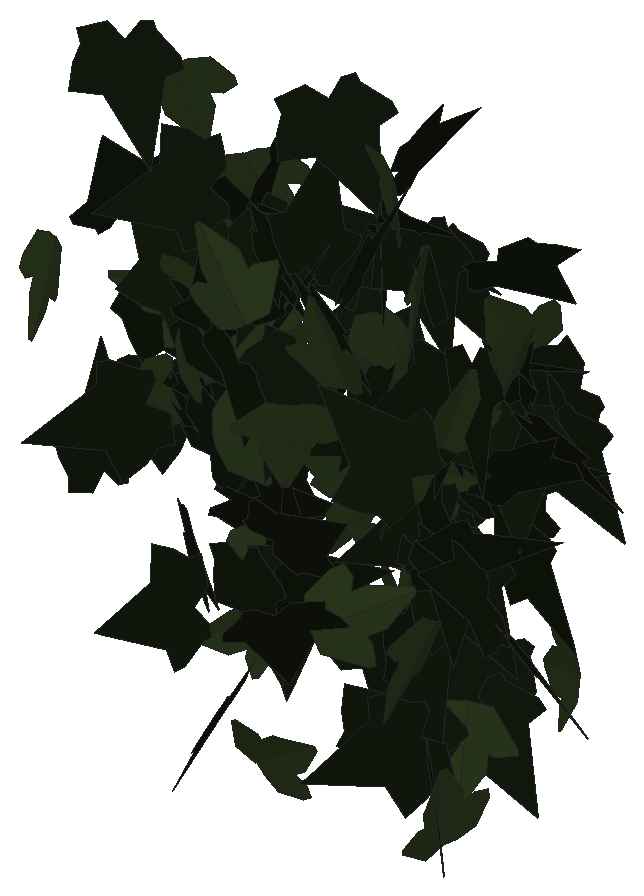
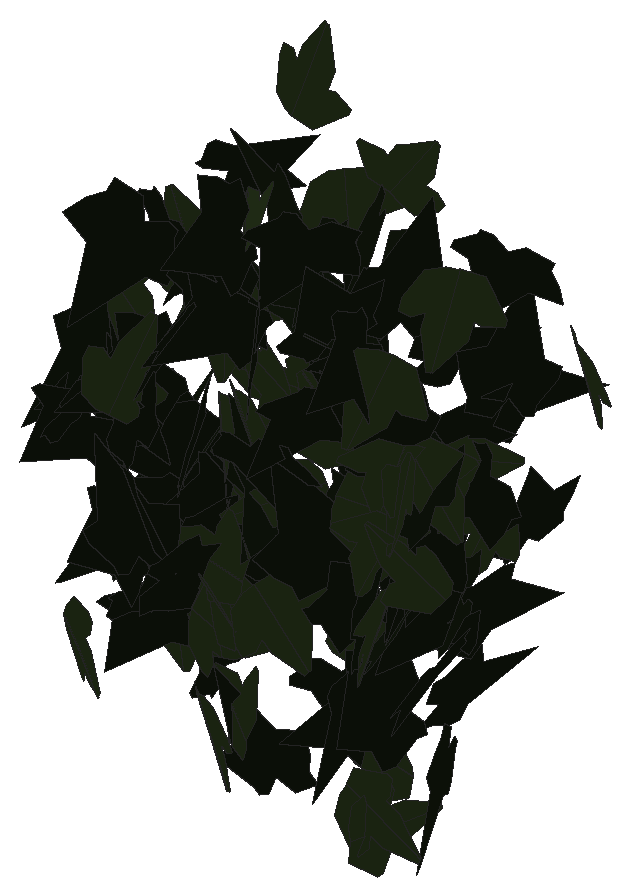
# SketchUp Ruby script. Lengths in inches.
U = 1.inch
M = Sketchup.active_model
def pt(a) = Geom::Point3d.new(a.map { |v| v * U })
def face(e, loops, mat)
  f = e.add_face(loops[0].map { |a| pt(a) })
  loops[1..].each { |l| e.add_face(l.map { |a| pt(a) }).erase! }
  f.material = f.back_material = mat if mat
  f
end
# faces: each face lists its corners as indices into pts; further lists are holes
def faces(e, pts, list, mat = nil) = list.each { |f| face(e, (f[0].is_a?(Array) ? f : [f]).map { |l| l.map { |i| pts[i] } }, mat) }
# xy, xz, yz: faces in a plane at the given z, y or x. An outline is a flat list of corners, or four numbers for a rectangle; further outlines are holes
def ring(l) = l.size == 4 ? [[l[0], l[1]], [l[2], l[1]], [l[2], l[3]], [l[0], l[3]]] : l.each_slice(2).to_a
def flat(e, list, mat, &to3) = list.each { |f| face(e, (f[0].is_a?(Array) ? f : [f]).map { |l| ring(l).map { |u, v| to3.(u, v) } }, mat) }
def xy(e, z, list, mat = nil) = flat(e, list, mat) { |x, y| [x, y, z] }
def xz(e, y, list, mat = nil) = flat(e, list, mat) { |x, z| [x, y, z] }
def yz(e, x, list, mat = nil) = flat(e, list, mat) { |y, z| [x, y, z] }
def lines(e, pts, list) = list.each { |a, b| e.add_line(pt(pts[a]), pt(pts[b])) }
# prism: a flat outline (further loops are holes) pulled along v
def prism(e, loops, v, mat = nil)
  f = face(e, loops, mat); d = Geom::Vector3d.new(v.map { |x| x * U })
  f.pushpull(f.normal.samedirection?(d) ? d.length : -d.length)
end
def box(e, o, s, mat = nil) = prism(e, [[o, [o[0] + s[0], o[1], o[2]], [o[0] + s[0], o[1] + s[1], o[2]], [o[0], o[1] + s[1], o[2]]]], [0, 0, s[2]], mat)
def at(x, y, z, deg = 0) = Geom::Transformation.translation(pt([x, y, z])) * Geom::Transformation.rotation(ORIGIN, Z_AXIS, deg.degrees)
def axes(o, x, y, z) = Geom::Transformation.new([*x, 0, *y, 0, *z, 0, *pt(o).to_a, 1])
def part(name) = M.definitions.add(name)
# library, detail: a bought-in or finely detailed component or shape, given as its bounding box
def library(name, o, s) = part(name).tap { |d| box(d.entities, o, s) }
def detail(e, o, s) = box(e.add_group.entities, o, s)
def put(e, d, t, mat = nil) = e.add_instance(d, t).tap { |i| i.material = mat if mat }
def group(e, t, mat = nil) = e.add_group.tap { |g| g.transformation = t; g.material = mat if mat }.entities
root = M.entities
M.materials.add("efeu1").color = [18, 25, 13]
M.materials.add("efeu2").color = [43, 57, 29]
c1 = part("ivyleaf_10")
p = [[0,0.5,-0.03],[-0.0625,2.02,-0.43],[-0.19,2.01,-0.46],[-0.54,1.05,-0.29],[-0.52,0.625,-0.18],[-0.83,0.76,-0.28],
  [-1.16,0.64,-0.33],[-1.15,0.33,-0.24],[-0.77,-0.39,0.02],[-0.3,-0.51,0.16],[0.04,-0.48,0.23],[-0.02,2.01,-0.4375],
  [-0.06,2.01,-0.43],[0.04,-0.49,0.23],[0.67,-0.49,0.14],[1.38,0.36,-0.2],[1.375,0.51,-0.24],[0.81,0.65,-0.19],
  [0.62,0.59,-0.15],[0.6,1.09,-0.28],[0.5,1.23,-0.31]]
faces(c1.entities,p,[[0,1,2,3,4,5,6,7,8,9,10],[11,12,0,13,14,15,16,17,18,19,20]],"efeu2")
c2 = part("ivyleaf_9")
p = [[1.54,2.16,1.25],[1.36,2.04,1.19],[-0.21,0.99,0.68],[-0.71,1.11,0.82],[-0.85,0.86,0.67],[-0.8,0.17,0.21],
  [-0.9,-0.01,0.1],[-0.67,-0.16,-0.02],[-0.08,-0.08,-0.05],[-0.03,-0.6,-0.4],[0.65,-0.88,-0.66],[0.83,-0.6,-0.49],
  [1.29,-0.42,-0.43],[1.8125,-0.07,-0.26],[1.21,0.44,0.15]]
faces(c2.entities,p,[[0,1,2,3,4,5,6,7,8,9,10,11,12,13,14]],"efeu1")
put(root,c1,axes([40.33,218.36,213.33],[-0.47908,0.07707,-0.12061],[-0.11885,0.0206,0.48523],[0.07976,0.49359,-0.00142]))
put(root,c2,axes([38.68,218.42,208.39],[-0.28519,0.35425,-0.20778],[0.13145,-0.16092,-0.45478],[-0.38909,-0.31402,-0.00135]))
put(root,c2,axes([39.54,218.27,209.85],[0.23659,0.41102,-0.15839],[-0.07808,-0.13781,-0.47425],[-0.43351,0.24914,-0.00102]))
put(root,c1,axes([39.57,218.5,212.375],[-0.35718,-0.34582,0.05319],[-0.03826,-0.03696,-0.49716],[0.34779,-0.35923,-0.00006]))
put(root,c2,axes([41.16,218.62,212.16],[-0.38091,-0.29363,-0.13671],[-0.10498,-0.08774,0.48092],[-0.30642,0.39507,0.00519]))
put(root,c1,axes([39.89,218.83,209.7],[0.19045,0.03633,-0.46088],[0.42264,0.18833,0.18949],[0.18736,-0.46175,0.04103]))
put(root,c2,axes([38.1,219.35,212.21],[0.0794,-0.37395,0.32227],[0.10808,-0.30532,-0.38092],[0.48168,0.13015,0.03234]))
put(root,c2,axes([38.89,219.07,210.3],[0.44987,0.09893,-0.1945],[0.17628,0.09792,0.45753],[0.12862,-0.48023,0.05322]))
put(root,c2,axes([36.62,219.41,211.12],[-0.06203,-0.20027,-0.45392],[-0.0142,-0.45655,0.20337],[-0.49593,0.03812,0.05095]))
put(root,c2,axes([38.28,219.23,209.67],[0.22042,-0.44879,-0.00135],[-0.00042,0.0013,-0.5],[0.44879,0.22042,0.0002]))
put(root,c1,axes([38.28,219.11,213.1875],[0.40005,0.11614,0.27654],[-0.26746,-0.07053,0.41652],[0.13576,-0.48118,0.00569]))
put(root,c1,axes([38.51,219.35,207.12],[-0.30257,-0.15729,0.36566],[0.38308,0.00974,0.32117],[-0.10815,0.47452,0.11462]))
put(root,c1,axes([40.93,219.64,206.94],[-0.11437,-0.4666,-0.13859],[-0.03341,-0.13451,0.48041],[-0.4856,0.11915,-0.00041]))
put(root,c2,axes([40.6,219.76,207.54],[0.05164,-0.03413,-0.49615],[0.47859,-0.1322,0.05891],[-0.13521,-0.481,0.01901]))
put(root,c1,axes([34.95,219.78,212.32],[0.40818,-0.28104,0.0664],[0.05534,-0.03672,-0.49557],[0.28342,0.41191,0.00113]))
put(root,c1,axes([40.27,220,209.06],[0.10747,-0.39995,0.28016],[0.06561,-0.27243,-0.4141],[0.48389,0.12577,-0.00607]))
put(root,c2,axes([40.05,220.18,207.61],[-0.01459,-0.19185,-0.4615],[-0.02795,-0.46066,0.19239],[-0.49901,0.03141,0.00272]))
put(root,c2,axes([39.55,219.96,211.81],[-0.36479,0.33876,0.04661],[-0.03452,0.03133,-0.49782],[-0.3402,-0.36642,0.00053]))
put(root,c2,axes([37.34,220.22,212.23],[0.34841,0.11708,0.33897],[-0.32039,-0.11071,0.36755],[0.16112,-0.47332,-0.00212]))
put(root,c1,axes([40.58,220.125,211.75],[-0.13186,-0.48078,0.03821],[0.02724,0.03213,0.49822],[-0.48153,0.13347,0.01772]))
put(root,c2,axes([35.64,219.95,209.77],[-0.19412,-0.30059,0.34923],[0.17924,0.29985,0.35772],[-0.42449,0.26407,-0.00866]))
put(root,c2,axes([40.21,220.58,212.0625],[0.1517,-0.3462,-0.32731],[0.13303,-0.29906,0.37798],[-0.45748,-0.20177,0.00137]))
put(root,c2,axes([38.04,220.55,211.625],[-0.12047,-0.47459,0.10127],[-0.02428,-0.09832,-0.48964],[0.48466,-0.12289,0.00065]))
put(root,c1,axes([39.98,220.23,211.56],[-0.3427,-0.36394,-0.01033],[0.0105,0.0043,-0.49987],[0.36393,-0.34283,0.0047]))
put(root,c2,axes([37.73,220.22,213.37],[0.35903,-0.16597,-0.30586],[-0.27385,0.13641,-0.39548],[0.21472,0.45149,0.00705]))
put(root,c2,axes([38.3125,220.47,212.65],[0.36198,-0.33394,0.08634],[0.06076,-0.06147,-0.49247],[0.33952,0.36703,-0.00392]))
put(root,c2,axes([40.6,220.73,209.41],[0.24364,-0.41487,-0.13609],[0.07452,-0.11405,0.48108],[-0.43022,-0.2547,0.00626]))
put(root,c2,axes([40.59,220.52,212.49],[-0.26539,-0.03778,-0.42207],[0.41667,0.06743,-0.26803],[0.07717,-0.49399,-0.0043]))
put(root,c2,axes([39.65,220.24,207.34],[-0.2955,-0.02523,0.40254],[0.40117,0.03316,0.29658],[-0.04166,0.49826,0.00065]))
put(root,c2,axes([36.22,220.82,207.71],[-0.16561,-0.17804,0.43689],[-0.23886,-0.36765,-0.24037],[0.40684,-0.28833,0.03672]))
put(root,c2,axes([38.9,220.36,213.03],[-0.11636,0.45709,0.16591],[0.02826,-0.16395,0.47151],[0.48545,0.11911,0.01232]))
put(root,c2,axes([40,220.82,209.57],[0.09942,-0.42642,0.24141],[0.06127,-0.23358,-0.43782],[0.48617,0.11664,0.00581]))
put(root,c1,axes([40.24,220.8,207.6],[0.46701,0.1783,0.01074],[0.00911,0.00625,-0.49988],[-0.17839,0.46709,0.00258]))
put(root,c1,axes([37.76,220.73,210.66],[-0.23216,-0.38234,0.22343],[0.11734,0.19014,0.4473],[-0.42701,0.26012,0.00144]))
put(root,c1,axes([36.78,220.9,210.12],[0.315,-0.11659,-0.37038],[0.35719,-0.10006,0.33527],[-0.1523,-0.47581,0.02025]))
put(root,c2,axes([37.78,220.49,212.12],[-0.26208,0.33166,-0.26705],[-0.16274,0.21176,0.4227],[0.39349,0.30848,-0.00305]))
put(root,c1,axes([35.58,220.68,210.35],[-0.04228,-0.34361,-0.36076],[0.11467,0.34562,-0.34263],[0.48483,-0.11171,0.04957]))
put(root,c2,axes([37.86,220.52,208.66],[0.01677,0.21115,-0.45292],[-0.07229,0.44943,0.20684],[0.49446,0.05854,0.0456]))
put(root,c2,axes([34.99,221.14,212.43],[0.24594,0.22385,0.37337],[-0.26973,-0.25825,0.3325],[0.3417,-0.36497,-0.00627]))
put(root,c2,axes([39.93,220.68,209.71],[0.1339,0.30022,-0.37675],[0.12607,0.35557,0.32814],[0.46495,-0.18287,0.01952]))
put(root,c2,axes([40.22,221.11,207.71],[-0.0968,-0.2891,-0.3963],[0.21187,0.33968,-0.29954],[0.44243,-0.22592,0.05674]))
put(root,c2,axes([40.66,221.125,208.73],[0.45015,-0.21747,-0.00843],[-0.00568,0.00763,-0.49991],[0.21756,0.45016,0.0044]))
put(root,c2,axes([35.85,221.56,212.77],[-0.23036,-0.17206,0.40906],[-0.30171,-0.27725,-0.28653],[0.32542,-0.37885,0.02391]))
put(root,c2,axes([39.78,221.21,209.3],[-0.13219,-0.17756,-0.44833],[0.3129,0.32213,-0.21984],[0.36691,-0.33868,0.02595]))
put(root,c2,axes([34.87,221.32,214.41],[-0.24398,-0.24467,-0.3614],[0.28442,0.22491,-0.34427],[0.33103,-0.37357,0.02943]))
put(root,c1,axes([38.26,221.43,211.5],[0.04633,-0.02596,-0.49717],[0.40135,-0.29349,0.05272],[-0.29457,-0.40397,-0.00636]))
put(root,c1,axes([35.83,221.34,211.39],[-0.04053,0.01498,-0.49813],[-0.49724,-0.03464,0.03942],[-0.03333,0.49857,0.0177]))
put(root,c2,axes([40.1,221.58,208.22],[-0.22659,-0.43668,0.08927],[-0.03559,-0.0821,-0.49193],[0.44429,-0.22929,0.00612]))
put(root,c2,axes([35.25,221.24,211.24],[-0.00289,-0.01896,-0.49963],[0.42273,0.26672,-0.01257],[0.267,-0.4225,0.01449]))
put(root,c2,axes([39.07,220.93,210.04],[0.00383,0.12453,0.48423],[-0.01252,0.48412,-0.1244],[-0.49983,-0.01117,0.00683]))
put(root,c1,axes([39.23,221.18,210.66],[0.15558,-0.38404,-0.27983],[-0.09853,0.26198,-0.41432],[0.46485,0.18406,0.00584]))
put(root,c2,axes([35.11,221.73,209.72],[0.0507,-0.19087,-0.45934],[0.11143,-0.44563,0.19747],[-0.48478,-0.1224,-0.00265]))
put(root,c2,axes([40.5625,221.02,210.88],[0.31687,0.22486,0.31469],[0.23653,0.20922,-0.38766],[-0.30602,0.39454,0.02622]))
put(root,c2,axes([35.78,221.43,211.64],[-0.35965,-0.34732,-0.0051],[-0.00315,-0.00408,0.49997],[-0.34734,0.35966,0.00074]))
put(root,c2,axes([37.22,221.11,210.08],[-0.11573,0.4522,0.17922],[-0.04368,0.17382,-0.46677],[-0.48446,-0.12369,-0.00073]))
put(root,c1,axes([38.41,221.74,213.5625],[-0.16663,-0.04986,0.46877],[0.38069,-0.30748,0.10262],[0.27805,0.39111,0.14044]))
put(root,c1,axes([38.9,221.67,212.73],[0.28997,-0.30876,0.26568],[0.20192,-0.17428,-0.42291],[0.35376,0.35256,0.02362]))
put(root,c2,axes([35.98,221.55,209.34],[-0.04118,0.01518,0.49807],[0.38457,-0.31684,0.04145],[0.31687,0.3865,0.01442]))
put(root,c1,axes([40.3125,221.73,212.19],[0.10972,-0.41494,0.25648],[0.07946,-0.24417,-0.42903],[0.4813,0.13491,0.01236]))
put(root,c2,axes([37.1,221.625,208.11],[-0.30782,-0.31398,-0.23804],[0.16263,0.17389,-0.43967],[0.35888,-0.34811,-0.00493]))
put(root,c2,axes([39.11,221.91,209.375],[0.02027,-0.25141,-0.43172],[0.01961,-0.43134,0.25211],[-0.4992,-0.02715,-0.00763]))
put(root,c2,axes([37.46,221.39,212.45],[-0.24975,-0.21038,0.37863],[0.28686,0.24716,0.32654],[-0.32456,0.38033,-0.00276]))
put(root,c2,axes([38.83,221.66,209.77],[0.04866,-0.04011,-0.49601],[0.48405,0.11943,0.03783],[0.11544,-0.48387,0.05046]))
put(root,c1,axes([37.85,221.4,210.22],[-0.13392,-0.11576,-0.46762],[0.40603,0.23406,-0.17422],[0.25923,-0.4264,0.03131]))
put(root,c1,axes([35.75,221.38,210.73],[-0.13919,0.28502,0.38651],[-0.17339,0.34544,-0.31718],[-0.44784,-0.22233,0.00267]))
put(root,c2,axes([40.2,221.86,211.04],[-0.20808,-0.40679,-0.20304],[0.09689,0.17848,-0.4569],[0.4442,-0.22949,0.00455]))
put(root,c2,axes([38.39,221.33,210.05],[0.01059,0.36168,0.34508],[0.01253,0.34485,-0.36183],[-0.49973,0.01631,-0.00176]))
put(root,c2,axes([39.02,222.04,210.83],[0.10162,-0.07137,-0.48433],[0.42022,-0.24107,0.12369],[-0.25117,-0.4322,0.01099]))
put(root,c2,axes([40.69,221.61,211.28],[0.49908,-0.02386,-0.01877],[-0.0184,0.00811,-0.4996],[0.02415,0.49936,0.00721]))
put(root,c2,axes([38.92,221.55,207.61],[-0.09533,-0.20801,0.44457],[0.20034,0.39695,0.22869],[-0.44808,0.22173,0.00767]))
put(root,c2,axes([35.1875,221.77,209.875],[0.41425,-0.27676,-0.04248],[-0.03064,0.03059,-0.49812],[0.27832,0.41529,0.00839]))
put(root,c1,axes([36.49,222.13,210.84],[-0.06993,-0.20984,0.44842],[-0.14264,-0.42513,-0.22118],[0.47409,-0.15886,-0.0004]))
put(root,c1,axes([35.32,221.77,213.96],[-0.3993,-0.281,-0.1077],[0.08788,0.06225,-0.48826],[0.28781,-0.40886,-0.00033]))
put(root,c2,axes([39.03,222.03,209.17],[0.06052,-0.49523,-0.03293],[-0.00349,0.03274,-0.49891],[0.49631,0.06062,0.00051]))
put(root,c2,axes([36.66,222.03,212.25],[-0.45598,-0.1113,-0.17232],[0.16661,0.04407,-0.46936],[0.11967,-0.48546,-0.0031]))
put(root,c2,axes([38.68,221.97,212.88],[-0.24987,-0.16759,-0.39934],[0.33372,0.21935,-0.30086],[0.27604,-0.41689,0.00224]))
put(root,c1,axes([38.32,221.95,211.42],[0.40211,-0.28,-0.09954],[-0.07615,0.06481,-0.4899],[0.28724,0.40915,0.00948]))
put(root,c2,axes([40.04,221.76,213.18],[0.34811,0.35097,0.0751],[0.05305,0.05316,-0.49433],[-0.35497,0.35213,-0.00023]))
put(root,c2,axes([37.29,222.05,214.17],[-0.12761,-0.29944,-0.37954],[0.15362,0.34708,-0.32548],[0.45839,-0.19968,0.00341]))
put(root,c2,axes([35.28,221.95,207.82],[0.31424,-0.10265,-0.37512],[-0.35728,0.11433,-0.33057],[0.15365,0.47581,-0.0015]))
put(root,c2,axes([35.12,222.38,211.4375],[0.38686,-0.12319,-0.29183],[0.27089,-0.11012,0.40558],[-0.1642,-0.47191,-0.01846]))
put(root,c2,axes([39.97,222.1875,209.25],[-0.07195,-0.02556,-0.49414],[0.4747,0.13731,-0.07622],[0.1396,-0.4801,0.0045]))
put(root,c2,axes([39.74,221.75,211.39],[0.24339,0.24344,0.36263],[0.25651,0.25632,-0.34424],[-0.3535,0.35361,-0.00012]))
put(root,c1,axes([35.89,222.19,207.54],[0.09164,-0.08342,-0.4844],[0.47239,-0.12123,0.11024],[-0.13584,-0.47785,0.05659]))
put(root,c1,axes([38.2,222.18,208.5],[-0.41891,-0.22532,0.15409],[0.14008,0.0648,0.47558],[-0.23429,0.44162,0.00884]))
put(root,c1,axes([37.7,222.33,209.16],[-0.22204,-0.37589,0.24372],[-0.12685,-0.20813,-0.43657],[0.42966,-0.25571,-0.00294]))
put(root,c2,axes([35.44,221.98,210.69],[0.45253,0.1469,-0.15375],[-0.14615,-0.04773,-0.47577],[-0.15446,0.47555,-0.00026]))
put(root,c2,axes([35.34,221.78,209.93],[0.23237,0.3735,0.2377],[0.10877,0.21207,-0.43954],[-0.42916,0.25598,0.01731]))
put(root,c1,axes([36.02,222.52,206.76],[0.01522,-0.00238,-0.49976],[-0.26236,-0.4256,-0.00596],[-0.42537,0.26241,-0.0142]))
put(root,c1,axes([35.42,222.31,211.77],[-0.34667,-0.23718,0.27123],[-0.20919,-0.17396,-0.41949],[0.29336,-0.40433,0.02138]))
put(root,c2,axes([35.75,222.26,211.99],[0.12415,-0.16427,0.45563],[0.42932,-0.18043,-0.18203],[0.22422,0.43642,0.09625]))
put(root,c2,axes([38.28,222.02,212.86],[0.47982,0.06395,0.12522],[0.1241,0.01672,-0.48407],[-0.0661,0.49561,0.00017]))
put(root,c1,axes([38.63,222.26,207.36],[0.38595,-0.31056,-0.06779],[-0.049,0.04723,-0.49535],[0.31407,0.389,0.00602]))
put(root,c2,axes([37.76,222.47,212.67],[-0.02622,0.02132,-0.49886],[0.46206,-0.1883,-0.03233],[-0.18925,-0.4627,-0.00983]))
put(root,c1,axes([38.4375,222.54,208.79],[0.06732,-0.35285,0.3478],[0.10035,-0.33401,-0.35828],[0.48518,0.11805,0.02584]))
put(root,c2,axes([37.66,222.23,206.86],[-0.22766,0.0804,0.43784],[0.37456,-0.23117,0.23721],[0.24057,0.436,0.04503]))
put(root,c2,axes([38.89,222.2,212.63],[0.25082,-0.34001,-0.26736],[-0.12808,0.23682,-0.42132],[0.41314,0.27984,0.0317]))
put(root,c2,axes([37.76,222.48,211.28],[-0.40164,-0.21857,-0.20227],[0.18413,0.08466,-0.45709],[0.23406,-0.44165,0.01249]))
put(root,c1,axes([37.9,222.49,207.53],[-0.17514,0.01873,0.46795],[0.44392,-0.15253,0.17225],[0.1492,0.4758,0.03679]))
put(root,c1,axes([36.01,222.25,212.8],[-0.43244,-0.18614,-0.16836],[0.15553,0.06449,-0.4708],[0.19699,-0.45956,0.00212]))
put(root,c2,axes([39.73,222.45,211.2],[-0.2516,-0.16245,-0.40038],[0.37572,0.14655,-0.29556],[0.21338,-0.44959,0.04832]))
put(root,c2,axes([39.4375,222.6,210.95],[-0.00135,-0.08215,0.4932],[0.23482,-0.43553,-0.0719],[0.44143,0.23144,0.03976]))
put(root,c2,axes([40.36,222.35,210.74],[-0.08774,-0.15417,-0.46748],[0.37051,0.29194,-0.16582],[0.32408,-0.3755,0.06301]))
put(root,c1,axes([35.84,222.26,210.73],[0.32304,0.31903,0.20943],[0.1493,0.14687,-0.45403],[-0.35121,0.35588,-0.00038]))
put(root,c2,axes([36.35,222.3,209.19],[0.0815,-0.29582,0.39478],[-0.06178,0.39086,0.30563],[-0.48943,-0.0986,0.02716]))
put(root,c2,axes([38.42,221.97,213.76],[0.11752,0.22342,0.43159],[0.16958,0.39727,-0.25183],[-0.45545,0.20557,0.0176]))
put(root,c2,axes([36.75,222.36,210.15],[0.33327,0.36468,0.07704],[-0.05428,-0.05476,0.49402],[0.36876,-0.33765,0.00309]))
put(root,c2,axes([40.28,222.83,211.1],[-0.12357,-0.34877,0.33629],[-0.12136,-0.31371,-0.36994],[0.46904,-0.17305,-0.00713]))
put(root,c1,axes([38.13,222.6,208.92],[0.10816,-0.19651,-0.44686],[0.36772,-0.26823,0.20696],[-0.32107,-0.37341,0.08649]))
put(root,c2,axes([39.84,222.28,209.88],[-0.15856,0.02252,-0.47366],[-0.47419,-0.00675,0.15842],[0.00074,0.49945,0.0235]))
put(root,c1,axes([35.64,222.38,211.86],[0.34066,0.33955,0.13659],[0.09764,0.09552,-0.48098],[-0.35273,0.35437,-0.00123]))
put(root,c1,axes([38.14,222.47,209.52],[-0.10232,-0.05793,0.48598],[0.48038,0.08308,0.11105],[-0.09361,0.48963,0.03866]))
put(root,c2,axes([39.46,222.53,209.35],[-0.24148,-0.0196,0.43738],[0.37193,-0.27272,0.19312],[0.231,0.41862,0.14629]))
put(root,c1,axes([40.61,222.27,207.77],[0.1468,-0.15526,-0.45204],[-0.30404,0.33454,-0.21364],[0.36879,0.33761,0.00381]))
put(root,c2,axes([36.83,222.38,212.15],[0.02835,-0.30201,-0.39747],[0.09536,0.39406,-0.29262],[0.49,-0.05921,0.07994]))
put(root,c1,axes([39.61,222.76,211.52],[-0.20066,-0.34278,-0.30371],[-0.15062,-0.26374,0.39718],[-0.43249,0.25089,0.00259]))
put(root,c2,axes([35.8,222.2,208.375],[0.35381,0.15279,0.31856],[0.29023,0.1314,-0.38536],[-0.20147,0.45759,0.00429]))
put(root,c2,axes([35.42,222.6,209.87],[0.27377,-0.4182,-0.01272],[-0.00699,0.01063,-0.49984],[0.41833,0.27386,-0.00002]))
put(root,c1,axes([36.11,222.56,207.16],[-0.2031,-0.01262,0.45672],[-0.44617,-0.10215,-0.20124],[0.09839,-0.48929,0.03023]))
put(root,c1,axes([35.9,222.38,209.79],[-0.16985,0.43928,0.16788],[-0.06714,0.15402,-0.47093],[-0.46545,-0.18252,0.00667]))
put(root,c2,axes([36.35,222.17,213.03],[-0.10736,0.19064,-0.44959],[-0.28558,0.3489,0.21614],[0.39613,0.3032,0.03396]))
put(root,c2,axes([38.68,222.99,209.44],[-0.0187,-0.34487,-0.36155],[0.01735,-0.36203,0.34443],[-0.49935,0.00034,0.0255]))
put(root,c1,axes([35.07,222.57,210.43],[0.30643,-0.0163,-0.39476],[0.39436,-0.01782,0.30686],[-0.02407,-0.49942,0.00194]))
put(root,c1,axes([35.5,222.51,211.76],[-0.40852,0.27709,0.0796],[-0.0729,0.03427,-0.49347],[-0.27892,-0.41479,0.0124]))
put(root,c2,axes([34.87,222.69,209.44],[0.20643,-0.43667,-0.12926],[-0.05436,0.11727,-0.483],[0.45214,0.21346,0.00094]))
put(root,c2,axes([36.37,222.34,208.33],[0.00444,0.02406,-0.4994],[-0.37002,0.33603,0.0129],[0.33625,0.36946,0.02079]))
